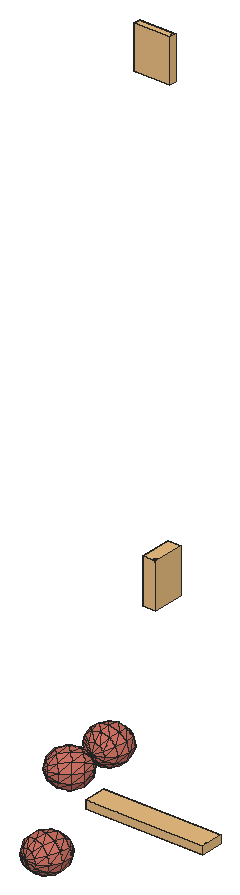
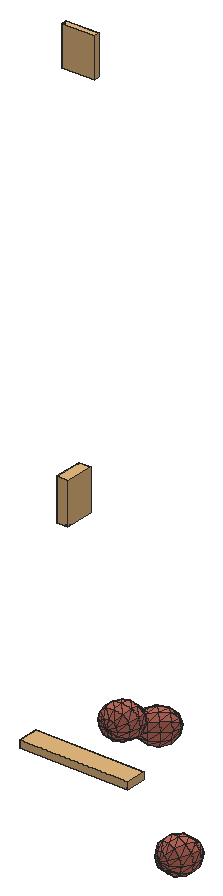
# SketchUp Ruby script. Lengths in inches.
U = 1.inch
M = Sketchup.active_model
def pt(a) = Geom::Point3d.new(a.map { |v| v * U })
def face(e, loops, mat)
  f = e.add_face(loops[0].map { |a| pt(a) })
  loops[1..].each { |l| e.add_face(l.map { |a| pt(a) }).erase! }
  f.material = f.back_material = mat if mat
  f
end
# faces: each face lists its corners as indices into pts; further lists are holes
def faces(e, pts, list, mat = nil) = list.each { |f| face(e, (f[0].is_a?(Array) ? f : [f]).map { |l| l.map { |i| pts[i] } }, mat) }
# xy, xz, yz: faces in a plane at the given z, y or x. An outline is a flat list of corners, or four numbers for a rectangle; further outlines are holes
def ring(l) = l.size == 4 ? [[l[0], l[1]], [l[2], l[1]], [l[2], l[3]], [l[0], l[3]]] : l.each_slice(2).to_a
def flat(e, list, mat, &to3) = list.each { |f| face(e, (f[0].is_a?(Array) ? f : [f]).map { |l| ring(l).map { |u, v| to3.(u, v) } }, mat) }
def xy(e, z, list, mat = nil) = flat(e, list, mat) { |x, y| [x, y, z] }
def xz(e, y, list, mat = nil) = flat(e, list, mat) { |x, z| [x, y, z] }
def yz(e, x, list, mat = nil) = flat(e, list, mat) { |y, z| [x, y, z] }
def lines(e, pts, list) = list.each { |a, b| e.add_line(pt(pts[a]), pt(pts[b])) }
# prism: a flat outline (further loops are holes) pulled along v
def prism(e, loops, v, mat = nil)
  f = face(e, loops, mat); d = Geom::Vector3d.new(v.map { |x| x * U })
  f.pushpull(f.normal.samedirection?(d) ? d.length : -d.length)
end
def box(e, o, s, mat = nil) = prism(e, [[o, [o[0] + s[0], o[1], o[2]], [o[0] + s[0], o[1] + s[1], o[2]], [o[0], o[1] + s[1], o[2]]]], [0, 0, s[2]], mat)
def at(x, y, z, deg = 0) = Geom::Transformation.translation(pt([x, y, z])) * Geom::Transformation.rotation(ORIGIN, Z_AXIS, deg.degrees)
def axes(o, x, y, z) = Geom::Transformation.new([*x, 0, *y, 0, *z, 0, *pt(o).to_a, 1])
def part(name) = M.definitions.add(name)
# library, detail: a bought-in or finely detailed component or shape, given as its bounding box
def library(name, o, s) = part(name).tap { |d| box(d.entities, o, s) }
def detail(e, o, s) = box(e.add_group.entities, o, s)
def put(e, d, t, mat = nil) = e.add_instance(d, t).tap { |i| i.material = mat if mat }
def group(e, t, mat = nil) = e.add_group.tap { |g| g.transformation = t; g.material = mat if mat }.entities
root = M.entities
M.materials.add("green").color = [174, 139, 102]
M.materials.add("vio").color = [206, 114, 100]
c1 = part("3DGeom~229_Defintion")
p = [[135.68,-61.63,-498.07],[-132.16,91.58,-492.59],[133.7,52.87,-500],[363.74,0,-373.43],[180.3,153.22,-454.61],[-51.45,265.375,-413.98],
  [185.71,-159.63,-449.34],[-128.73,-106.76,-489.25],[-362.61,105.75,-353.2],[-269.41,306.43,-262.42],[-269.41,306.43,-262.42],[-42.08,-276.49,-404.84],
  [-358.65,-123.27,-349.34],[262.99,212.5,-374.0625],[91.78,368.07,-274.47],[91.78,368.07,-274.47],[270.39,-214.85,-366.86],[-51.45,265.375,-413.98],
  [-269.41,306.43,-262.42],[-104.02,425.01,-101.32],[-51.45,265.375,-413.98],[91.78,368.07,-274.47],[104.59,-372.13,-261.99],[-258.59,-319.26,-251.875],
  [-42.08,-276.49,-404.84],[104.59,-372.13,-261.99],[-258.59,-319.26,-251.875],[359.62,214.85,-279.94],[262.99,212.5,-374.0625],[259.15,372.13,-111.44],
  [262.99,212.5,-374.0625],[259.15,372.13,-111.44],[359.62,214.85,-279.94],[367.02,-212.5,-272.74],[449.71,-153.21,-192.19],[367.02,-212.5,-272.74],
  [363.74,0,-373.43],[496.3125,-52.87,-146.8],[363.74,0,-373.43],[494.33,61.64,-148.73],[363.74,0,-373.43],[359.62,214.85,-279.94],
  [444.3,159.63,-197.46],[363.74,0,-373.43],[363.74,0,-373.43],[367.02,-212.5,-272.74],[104.59,-372.13,-261.99],[270.39,-214.85,-366.86],
  [-358.65,-123.27,-349.34],[-495.9,91.58,-119.16],[-362.61,105.75,-353.2],[-362.61,105.75,-353.2],[-415.1875,265.38,-40.55],[-362.61,105.75,-353.2],
  [-415.1875,265.38,-40.55],[-269.41,306.43,-262.42],[-258.59,-319.26,-251.875],[-492.47,-106.76,-115.82],[-358.65,-123.27,-349.34],[-358.65,-123.27,-349.34],
  [405.8125,276.49,31.41],[259.15,372.13,-111.44],[89.24,429.7,86.92],[259.15,372.13,-111.44],[367.02,-212.5,-272.74],[271.96,-368.07,-98.97],
  [104.59,-372.13,-261.99],[271.96,-368.07,-98.97],[367.02,-212.5,-272.74],[-415.1875,265.38,-40.55],[-271.96,368.07,98.97],[104.59,-372.13,-261.99],
  [-89.24,-429.7,-86.92],[-258.59,-319.26,-251.875],[104.59,-372.13,-261.99],[-405.8125,-276.49,-31.41],[-258.59,-319.26,-251.875],[-258.59,-319.26,-251.875],
  [-405.8125,-276.49,-31.41],[492.47,106.75,115.82],[415.1875,-265.375,40.55],[271.96,-368.07,-98.97],[495.9,-91.58,119.16],[-496.3125,52.87,146.8],
  [-449.71,153.21,192.19],[-415.1875,265.38,-40.55],[-494.33,-61.64,148.73],[259.15,372.13,-111.44],[258.59,319.26,251.875],[405.8125,276.49,31.41],
  [259.15,372.13,-111.44],[258.59,319.26,251.875],[-104.59,372.13,261.99],[104.02,-425.01,101.32],[415.1875,-265.375,40.55],[-259.15,-372.13,111.44],
  [-405.8125,-276.49,-31.41],[-415.1875,265.38,-40.55],[-367.02,212.5,272.74],[-415.1875,265.38,-40.55],[-367.02,212.5,272.74],[-271.96,368.07,98.97],
  [-259.15,-372.13,111.44],[-444.3,-159.63,197.46],[358.65,123.27,349.34],[258.59,319.26,251.875],[415.1875,-265.375,40.55],[269.41,-306.43,262.42],
  [269.41,-306.43,262.42],[42.08,276.49,404.84],[42.08,276.49,404.84],[258.59,319.26,251.875],[-367.02,212.5,272.74],[-270.39,214.85,366.86],
  [-270.39,214.85,366.86],[-91.78,-368.07,274.47],[-259.15,-372.13,111.44],[-359.62,-214.85,279.94],[-359.62,-214.85,279.94],[362.61,-105.75,353.2],
  [269.41,-306.43,262.42],[-363.74,0,373.43],[-367.02,212.5,272.74],[258.59,319.26,251.875],[42.08,276.49,404.84],[128.73,106.76,489.25],
  [258.59,319.26,251.875],[358.65,123.27,349.34],[-104.59,372.13,261.99],[-270.39,214.85,366.86],[-185.71,159.63,449.34],[-104.59,372.13,261.99],
  [51.45,-265.375,413.98],[362.61,-105.75,353.2],[51.45,-265.375,413.98],[269.41,-306.43,262.42],[-367.02,212.5,272.74],[-363.74,0,373.43],
  [-262.99,-212.5,374.0625],[-359.62,-214.85,279.94],[51.45,-265.375,413.98],[-262.99,-212.5,374.0625],[-91.78,-368.07,274.47],[-359.62,-214.85,279.94],
  [-262.99,-212.5,374.0625],[-363.74,0,373.43],[358.65,123.27,349.34],[132.16,-91.58,492.59],[362.61,-105.75,353.2],[358.65,123.27,349.34],
  [362.61,-105.75,353.2],[51.45,-265.375,413.98],[-363.74,0,373.43],[-262.99,-212.5,374.0625],[-180.3,-153.22,454.61],[-363.74,0,373.43],
  [-133.7,-52.87,500],[-363.74,0,373.43],[-135.68,61.63,498.07],[-363.74,0,373.43],[-363.74,0,373.43],[51.45,-265.375,413.98],
  [-262.99,-212.5,374.0625],[51.45,-265.375,413.98]]
faces(c1.entities,p,[[0,1,2],[0,2,3],[2,4,3],[2,1,5],[2,5,4],[6,7,0],[6,0,3],[0,7,1],
  [7,8,1],[1,8,9],[1,10,5],[11,12,7],[6,11,7],[7,12,8],[4,13,3],[4,5,14],
  [4,15,13],[16,11,6],[16,6,3],[17,18,19],[20,19,21],[22,23,24],[16,25,11],[11,26,12],
  [13,27,3],[28,21,29],[30,31,32],[33,16,3],[34,35,36],[37,34,38],[39,37,40],[41,42,43],
  [42,39,44],[45,46,47],[48,49,50],[51,49,52],[53,54,55],[56,57,58],[59,57,49],[41,60,42],
  [41,61,60],[21,19,62],[21,62,63],[64,65,66],[34,67,68],[18,69,70],[18,70,19],[71,72,73],
  [65,72,74],[72,75,76],[77,78,57],[42,79,39],[42,60,79],[34,80,81],[37,80,34],[39,79,82],
  [39,82,37],[37,82,80],[57,83,49],[49,83,84],[49,84,85],[78,86,57],[57,86,83],[87,88,89],
  [90,62,91],[19,70,92],[19,92,62],[65,93,72],[94,93,65],[72,95,96],[93,95,72],[97,84,98],
  [99,100,101],[102,103,78],[78,103,86],[60,104,79],[60,105,104],[106,107,93],[82,108,80],[62,92,109],
  [62,110,111],[70,112,113],[70,114,92],[93,115,95],[107,115,93],[116,117,103],[115,118,95],[79,104,119],
  [79,119,82],[82,119,120],[83,86,121],[84,83,121],[86,103,121],[122,84,121],[103,117,121],[123,124,125],
  [126,125,127],[128,129,130],[131,130,124],[107,132,115],[133,134,135],[129,136,137],[115,138,139],[140,141,142],
  [143,144,145],[146,147,148],[149,125,147],[150,147,151],[130,129,152],[153,154,155],[154,156,157],[156,158,159],
  [158,130,160],[161,154,162],[124,130,158],[124,158,125],[147,154,163],[147,156,154],[125,156,147],[125,158,156]],"vio")
c2 = library("3DGeom~19_Defintion",[-341.38,-500,-142.11],[682.76,1000,284.22])
c3 = part("3DGeom~20_Defintion")
p = [[-311.06,-487.18,-72.26],[-310.25,-484.5,-142.11],[-284.25,-498.77,-90.07],[-284.25,-498.77,-90.07],[-310.25,-484.5,-142.11],[-283.85,-497.43,-124.99],
  [-310.25,-484.5,-142.11],[-294.95,-491.76,-137.63],[-283.85,-497.43,-124.99],[-337.46,-474.24,-89.375],[-310.25,-484.5,-142.11],[-311.06,-487.18,-72.26],
  [-337.0625,-472.9,-124.3],[-310.25,-484.5,-142.11],[-337.46,-474.24,-89.375],[-310.25,-484.5,-142.11],[-337.0625,-472.9,-124.3],[-325.67,-477.6,-137.23],
  [-284.25,-498.77,-90.07],[-283.85,-497.43,-124.99],[-279.93,-500,-107.58],[-337.0625,-472.9,-124.3],[-337.46,-474.24,-89.375],[-341.38,-471.67,-106.78],
  [-311.06,-487.18,-72.26],[-284.25,-498.77,-90.07],[-295.64,-494.08,-77.14],[-337.46,-474.24,-89.375],[-311.06,-487.18,-72.26],[-326.37,-479.92,-76.74],
  [319.0625,494.74,82.9],[301.91,466.72,142.11],[318.42,461.52,137.94],[319.0625,494.74,82.9],[318.42,461.52,137.94],[332.8,461.46,126.96],
  [319.0625,494.74,82.9],[332.8,461.46,126.96],[341.21,466.57,112.1],[319.0625,494.74,82.9],[341.21,466.57,112.1],[341.38,475.47,97.35],
  [319.0625,494.74,82.9],[287.69,475.68,138.34],[301.91,466.72,142.11],[319.0625,494.74,82.9],[341.38,475.47,97.35],[333.27,485.79,86.67],
  [319.0625,494.74,82.9],[279.59,485.99,127.65],[287.69,475.68,138.34],[319.0625,494.74,82.9],[279.76,494.89,112.9],[279.59,485.99,127.65],
  [319.0625,494.74,82.9],[288.17,500,98.05],[279.76,494.89,112.9],[319.0625,494.74,82.9],[302.55,499.95,87.06],[288.17,500,98.05]]
faces(c3.entities,p,[[0,1,2],[3,4,5],[6,7,8],[9,10,11],[12,13,14],[15,16,17],[18,19,20],[21,22,23],
  [24,25,26],[27,28,29],[30,31,32],[33,34,35],[36,37,38],[39,40,41],[42,43,44],[45,46,47],
  [48,49,50],[51,52,53],[54,55,56],[57,58,59]],"green")
c4 = part("3DGeom~196_Defintion")
p = [[141.97,-189.5,-442.47],[-141.24,0,-495.8],[125.58,0,-500],[368.22,-109.41,-337.01],[368.22,-109.41,-337.01],[358.76,0,-370.22],
  [-122.32,218.8125,-429.38],[141.97,189.5,-442.47],[358.76,0,-370.22],[-122.32,-218.81,-429.38],[-370.22,0,-358.76],[-353.83,189.5,-301.23],
  [186.74,-328.22,-285.3125],[394.07,-189.5,-246.27],[394.07,-189.5,-246.27],[368.22,-109.41,-337.01],[358.76,0,-370.22],[368.22,109.41,-337.01],
  [368.22,109.41,-337.01],[186.74,328.22,-285.3125],[-70.62,378.99,-247.9],[-70.62,378.99,-247.9],[186.74,328.22,-285.3125],[-70.62,-378.99,-247.9],
  [-353.83,-189.5,-301.23],[-309.0625,328.22,-144.07],[-309.0625,328.22,-144.07],[-70.62,378.99,-247.9],[368.22,-109.41,-337.01],[358.76,0,-370.22],
  [495.8,0,-141.24],[368.22,109.41,-337.01],[-353.83,-189.5,-301.23],[-500,0,-125.58],[-370.22,0,-358.76],[-370.22,0,-358.76],
  [-490.54,109.41,-92.37],[-370.22,0,-358.76],[-353.83,189.5,-301.23],[394.07,-189.5,-246.27],[394.07,189.5,-246.27],[368.22,109.41,-337.01],
  [186.74,328.22,-285.3125],[394.07,189.5,-246.27],[-309.0625,-328.22,-144.07],[-309.0625,-328.22,-144.07],[-490.54,-109.41,-92.37],[-353.83,-189.5,-301.23],
  [-353.83,-189.5,-301.23],[-353.83,189.5,-301.23],[-464.6875,189.5,-1.63],[-353.83,189.5,-301.23],[-309.0625,328.22,-144.07],[247.9,-378.99,-70.62],
  [-70.62,-378.99,-247.9],[186.74,-328.22,-285.3125],[429.38,-218.8125,-122.32],[247.9,-378.99,-70.62],[186.74,-328.22,-285.3125],[186.74,-328.22,-285.3125],
  [186.74,328.22,-285.3125],[247.9,378.99,-70.62],[186.74,328.22,-285.3125],[-70.62,378.99,-247.9],[0,437.625,0],[186.74,328.22,-285.3125],
  [247.9,378.99,-70.62],[0,-437.625,0],[-309.0625,-328.22,-144.07],[-70.62,-378.99,-247.9],[247.9,-378.99,-70.62],[-70.62,-378.99,-247.9],
  [-309.0625,328.22,-144.07],[-247.9,378.99,70.62],[429.38,218.8125,-122.32],[-247.9,-378.99,70.62],[-309.0625,-328.22,-144.07],[-247.9,-378.99,70.62],
  [-464.6875,-189.5,-1.63],[-309.0625,-328.22,-144.07],[-309.0625,-328.22,-144.07],[-309.0625,328.22,-144.07],[-429.38,218.8125,122.32],[-309.0625,328.22,-144.07],
  [-247.9,378.99,70.62],[464.6875,-189.5,1.63],[490.54,-109.41,92.37],[500,0,125.58],[464.6875,189.5,1.63],[490.54,109.41,92.37],
  [-495.8,0,141.24],[309.0625,328.22,144.07],[309.0625,-328.22,144.07],[247.9,-378.99,-70.62],[309.0625,-328.22,144.07],[247.9,378.99,-70.62],
  [70.62,378.99,247.9],[309.0625,328.22,144.07],[247.9,378.99,-70.62],[70.62,378.99,247.9],[-247.9,-378.99,70.62],[-429.38,-218.8125,122.32],
  [70.62,-378.99,247.9],[309.0625,-328.22,144.07],[-186.74,328.22,285.3125],[-186.74,328.22,285.3125],[70.62,378.99,247.9],[353.83,189.5,301.23],
  [-186.74,-328.22,285.3125],[-247.9,-378.99,70.62],[-186.74,-328.22,285.3125],[-247.9,378.99,70.62],[-394.07,189.5,246.27],[-247.9,378.99,70.62],
  [-394.07,189.5,246.27],[-186.74,328.22,285.3125],[353.83,-189.5,301.23],[370.22,0,358.76],[-186.74,-328.22,285.3125],[-394.07,-189.5,246.27],
  [-394.07,189.5,246.27],[-368.22,-109.41,337.01],[-368.22,-109.41,337.01],[-358.76,0,370.22],[-358.76,0,370.22],[-368.22,109.41,337.01],
  [-368.22,109.41,337.01],[-394.07,189.5,246.27],[353.83,-189.5,301.23],[70.62,-378.99,247.9],[309.0625,-328.22,144.07],[309.0625,328.22,144.07],
  [122.32,218.8125,429.38],[353.83,189.5,301.23],[309.0625,328.22,144.07],[70.62,378.99,247.9],[-141.97,-189.5,442.47],[-394.07,-189.5,246.27],
  [-186.74,-328.22,285.3125],[-368.22,-109.41,337.01],[-394.07,-189.5,246.27],[-186.74,328.22,285.3125],[-394.07,189.5,246.27],[-368.22,109.41,337.01],
  [122.32,-218.8125,429.38],[-186.74,-328.22,285.3125],[70.62,-378.99,247.9],[353.83,-189.5,301.23],[70.62,-378.99,247.9],[-141.97,189.5,442.47],
  [-186.74,-328.22,285.3125],[370.22,0,358.76],[353.83,-189.5,301.23],[353.83,189.5,301.23],[141.24,0,495.8],[353.83,189.5,301.23],
  [370.22,0,358.76],[-125.58,0,500],[-358.76,0,370.22],[370.22,0,358.76]]
faces(c4.entities,p,[[0,1,2],[3,0,2],[4,2,5],[2,1,6],[2,6,7],[8,2,7],[9,10,1],[0,9,1],
  [1,10,11],[1,11,6],[12,9,0],[13,12,0],[14,0,15],[16,7,17],[18,7,19],[7,6,20],
  [7,21,22],[23,24,9],[12,23,9],[9,24,10],[6,11,25],[6,26,27],[28,29,30],[29,31,30],
  [32,33,34],[35,33,36],[37,36,38],[39,28,30],[31,40,30],[41,42,43],[23,44,24],[45,46,47],
  [48,46,33],[49,36,50],[51,50,52],[53,54,55],[56,57,58],[56,59,39],[40,60,61],[62,63,64],
  [65,64,66],[67,68,69],[70,67,71],[63,72,73],[63,73,64],[56,39,30],[40,74,30],[40,61,74],
  [67,75,76],[77,78,79],[80,78,46],[81,50,82],[83,82,84],[85,56,30],[86,85,30],[87,86,30],
  [74,88,30],[88,89,30],[89,87,30],[33,46,90],[36,33,90],[85,57,56],[74,91,88],[74,61,91],
  [46,78,90],[50,36,90],[92,67,93],[85,94,57],[95,96,97],[98,64,99],[100,101,78],[78,101,90],
  [82,50,90],[102,75,67],[103,102,67],[64,73,104],[64,105,106],[86,94,85],[88,107,89],[88,91,107],
  [108,101,109],[102,110,75],[111,82,112],[113,114,115],[86,116,94],[87,116,86],[89,107,117],[89,117,87],
  [118,119,101],[101,119,90],[120,82,90],[87,117,116],[119,121,90],[122,123,90],[124,125,90],[126,127,90],
  [128,129,130],[131,132,133],[134,135,132],[136,137,138],[136,139,140],[141,142,143],[144,145,146],[147,144,148],
  [135,141,149],[135,149,132],[144,136,150],[141,143,149],[151,144,152],[153,132,154],[155,154,156],[157,139,136],
  [157,158,139],[149,143,158],[159,154,144],[149,158,157],[154,136,144],[132,149,157],[132,157,154],[154,157,136]],"vio")
c5 = library("3DGeom~27_Defintion",[-78.21,-500,-418.56],[156.42,1000,837.12])
c6 = part("3DGeom~28_Defintion")
p = [[46.32,-458.84,-418.56],[37.22,-500,-363.86],[12.49,-468.47,-409.44],[75.6,-469.79,-400.32],[37.22,-500,-363.86],[75.6,-469.79,-400.32],
  [63.93,-461.98,-412.26],[12.49,-468.47,-409.44],[27.49,-461.21,-417.52],[12.49,-468.47,-409.44],[37.22,-500,-363.86],[7.94,-489.05,-382.09],
  [12.49,-468.47,-409.44],[7.94,-489.05,-382.09],[5.33,-478.66,-396.47],[71.06,-490.37,-372.98],[37.22,-500,-363.86],[75.6,-469.79,-400.32],
  [71.06,-490.37,-372.98],[75.6,-469.79,-400.32],[78.21,-480.18,-385.94],[37.22,-500,-363.86],[19.61,-496.86,-370.16],[7.94,-489.05,-382.09],
  [37.22,-500,-363.86],[71.06,-490.37,-372.98],[56.05,-497.625,-364.89],[-47.11,487.39,418.56],[-36.4375,500,347.21],[-55.37,499.54,349.35],
  [-47.11,487.39,418.56],[-18.93,498.77,354.62],[-36.4375,500,347.21],[-47.11,487.39,418.56],[-55.37,499.54,349.35],[-70.66,497.51,360.48],
  [-47.11,487.39,418.56],[-7.55,496.1875,369.6],[-18.93,498.77,354.62],[-47.11,487.39,418.56],[-70.66,497.51,360.48],[-78.21,494.45,377.62],
  [-47.11,487.39,418.56],[-5.33,492.93,388.15],[-7.55,496.1875,369.6],[-47.11,487.39,418.56],[-78.21,494.45,377.62],[-76,491.2,396.16],
  [-47.11,487.39,418.56],[-12.88,489.88,405.28],[-5.33,492.93,388.15],[-47.11,487.39,418.56],[-76,491.2,396.16],[-64.61,488.61,411.15],
  [-47.11,487.39,418.56],[-28.17,487.85,416.41],[-12.88,489.88,405.28]]
faces(c6.entities,p,[[0,1,2],[3,4,0],[5,0,6],[0,7,8],[9,10,11],[12,13,14],[15,16,17],[18,19,20],
  [21,22,23],[24,25,26],[27,28,29],[30,31,32],[33,34,35],[36,37,38],[39,40,41],[42,43,44],
  [45,46,47],[48,49,50],[51,52,53],[54,55,56]],"green")
c7 = library("3DGeom~15_Defintion",[-93.43,-35.39,-500],[186.86,70.78,1000])
c8 = part("3DGeom~16_Defintion")
p = [[-67.78,-34.5625,-497.5],[-75.6,-25.33,-500],[-54.89,-33.15,-493.42],[-75.6,-25.33,-500],[-67.78,-34.5625,-497.5],[-73.08,-30.88,-499.18],
  [-54.89,-33.15,-493.42],[-75.6,-25.33,-500],[-49.81,-22.5,-491.85],[-75.6,-25.33,-500],[-74.66,-19.4,-499.72],[-70.52,-14.68,-498.43],
  [-57.625,-13.26,-494.36],[-75.6,-25.33,-500],[-70.52,-14.68,-498.43],[-49.81,-22.5,-491.85],[-75.6,-25.33,-500],[-57.625,-13.26,-494.36],
  [-57.625,-13.26,-494.36],[-70.52,-14.68,-498.43],[-64.28,-12.43,-496.47],[-67.78,-34.5625,-497.5],[-54.89,-33.15,-493.42],[-61.125,-35.39,-495.39],
  [-49.81,-22.5,-491.85],[-57.625,-13.26,-494.36],[-52.33,-16.95,-492.67],[-54.89,-33.15,-493.42],[-49.81,-22.5,-491.85],[-50.75,-28.42,-492.13],
  [67.2,22.73,500],[92.46,19.2,493.88],[93.43,25.1,493.15],[67.2,22.73,500],[93.43,25.1,493.15],[90.88,30.68,493.34],
  [67.2,22.73,500],[90.88,30.68,493.34],[85.51,34.45,494.39],[67.2,22.73,500],[88.24,14.5625,495.33],[92.46,19.2,493.88],
  [67.2,22.73,500],[85.51,34.45,494.39],[78.74,35.39,496.03],[67.2,22.73,500],[81.9,12.43,497.11],[88.24,14.5625,495.33],
  [67.2,22.73,500],[78.74,35.39,496.03],[72.39,33.26,497.82],[67.2,22.73,500],[75.13,13.38,498.76],[81.9,12.43,497.11],
  [67.2,22.73,500],[72.39,33.26,497.82],[68.17,28.625,499.27],[67.2,22.73,500],[69.75,17.15,499.8125],[75.13,13.38,498.76]]
faces(c8.entities,p,[[0,1,2],[3,4,5],[6,7,8],[9,10,11],[12,13,14],[15,16,17],[18,19,20],[21,22,23],
  [24,25,26],[27,28,29],[30,31,32],[33,34,35],[36,37,38],[39,40,41],[42,43,44],[45,46,47],
  [48,49,50],[51,52,53],[54,55,56],[57,58,59]],"green")
c9 = part("3DGeom~188_Defintion")
p = [[-5.63,-212.24,-433.01],[-255.63,0,-429.76],[-6.51,0,-500],[245.12,-183.8,-378.25],[244.37,0,-436.27],[-254.88,183.8,-371.75],
  [-5.63,212.24,-433.01],[430.2,-106.12,-222.14],[430.2,-106.12,-222.14],[429.76,0,-255.63],[245.12,183.8,-378.25],[429.76,0,-255.63],
  [245.12,183.8,-378.25],[-3.25,-367.61,-250],[-254.88,-183.8,-371.75],[247.18,-318.36,-219.76],[247.18,-318.36,-219.76],[-252.82,318.36,-213.25],
  [245.12,183.8,-378.25],[-3.25,367.61,-250],[-252.82,318.36,-213.25],[-3.25,367.61,-250],[-254.88,-183.8,-371.75],[-436.27,0,-244.37],
  [-255.63,0,-429.76],[-255.63,0,-429.76],[-435.83,106.12,-210.87],[-255.63,0,-429.76],[-254.88,183.8,-371.75],[431.39,-183.8,-130.63],
  [247.18,-318.36,-219.76],[245.12,-183.8,-378.25],[245.12,-183.8,-378.25],[430.2,-106.12,-222.14],[429.76,0,-255.63],[245.12,183.8,-378.25],
  [430.2,106.12,-222.14],[430.2,106.12,-222.14],[245.12,183.8,-378.25],[247.18,318.36,-219.76],[245.12,183.8,-378.25],[-3.25,367.61,-250],
  [247.18,318.36,-219.76],[-252.82,-318.36,-213.25],[-252.82,-318.36,-213.25],[-435.83,-106.12,-210.87],[-254.88,-183.8,-371.75],[-254.88,-183.8,-371.75],
  [-254.88,183.8,-371.75],[-434.64,183.8,-119.36],[-254.88,183.8,-371.75],[-252.82,318.36,-213.25],[429.76,0,-255.63],[500,0,-6.51],
  [0,-424.48,0],[-252.82,-318.36,-213.25],[-3.25,-367.61,-250],[250,-367.61,-3.25],[-3.25,-367.61,-250],[250,-367.61,-3.25],
  [-3.25,-367.61,-250],[247.18,-318.36,-219.76],[-3.25,367.61,-250],[-252.82,318.36,-213.25],[-250,367.61,3.25],[247.18,318.36,-219.76],
  [0,424.48,0],[-500,0,6.51],[431.39,183.8,-130.63],[433.01,-212.24,-5.63],[250,-367.61,-3.25],[250,367.61,-3.25],
  [247.18,318.36,-219.76],[250,367.61,-3.25],[-250,-367.61,3.25],[-252.82,-318.36,-213.25],[-250,-367.61,3.25],[-434.64,-183.8,-119.37],
  [-252.82,-318.36,-213.25],[-252.82,-318.36,-213.25],[-252.82,318.36,-213.25],[-433.01,212.24,5.63],[-252.82,318.36,-213.25],[-250,367.61,3.25],
  [433.01,212.24,-5.63],[-250,-367.61,3.25],[-433.01,-212.24,5.63],[434.64,-183.8,119.37],[435.83,-106.12,210.87],[436.27,0,244.37],
  [434.64,183.8,119.37],[435.83,106.12,210.87],[252.82,318.36,213.25],[252.82,-318.36,213.25],[250,-367.61,-3.25],[252.82,-318.36,213.25],
  [250,367.61,-3.25],[3.25,367.61,250],[252.82,318.36,213.25],[250,367.61,-3.25],[3.25,367.61,250],[3.25,-367.61,250],
  [252.82,-318.36,213.25],[-247.18,318.36,219.76],[-247.18,318.36,219.76],[3.25,367.61,250],[-247.18,-318.36,219.76],[-250,-367.61,3.25],
  [-247.18,-318.36,219.76],[-250,367.61,3.25],[-431.39,183.8,130.63],[-250,367.61,3.25],[-247.18,318.36,219.76],[-247.18,-318.36,219.76],
  [-431.39,-183.8,130.63],[-430.2,-106.12,222.14],[-429.76,0,255.63],[-429.76,0,255.63],[-430.2,106.12,222.14],[-430.2,106.12,222.14],
  [254.88,183.8,371.75],[-245.12,-183.8,378.25],[-247.18,-318.36,219.76],[-245.12,-183.8,378.25],[-247.18,318.36,219.76],[-430.2,106.12,222.14],
  [254.88,-183.8,371.75],[255.63,0,429.76],[254.88,-183.8,371.75],[3.25,-367.61,250],[252.82,-318.36,213.25],[252.82,318.36,213.25],
  [5.63,212.24,433.01],[254.88,183.8,371.75],[252.82,318.36,213.25],[3.25,367.61,250],[5.63,-212.24,433.01],[-247.18,-318.36,219.76],
  [3.25,-367.61,250],[-245.12,-183.8,378.25],[-247.18,-318.36,219.76],[-247.18,318.36,219.76],[-430.2,106.12,222.14],[-245.12,183.8,378.25],
  [-247.18,318.36,219.76],[-245.12,183.8,378.25],[-244.37,0,436.27],[-430.2,-106.12,222.14],[-429.76,0,255.63],[-430.2,-106.12,222.14],
  [-430.2,106.12,222.14],[254.88,-183.8,371.75],[3.25,-367.61,250],[255.63,0,429.76],[254.88,-183.8,371.75],[254.88,183.8,371.75],
  [6.51,0,500],[254.88,183.8,371.75],[255.63,0,429.76],[255.63,0,429.76]]
faces(c9.entities,p,[[0,1,2],[3,0,2],[3,2,4],[2,1,5],[2,5,6],[4,2,6],[7,3,4],[8,4,9],
  [4,6,10],[11,4,12],[13,14,0],[15,13,0],[16,0,3],[0,14,1],[6,5,17],[18,6,19],
  [6,20,21],[22,23,24],[25,23,26],[27,26,28],[29,30,31],[29,32,33],[34,35,36],[37,38,39],
  [40,41,42],[13,43,14],[44,45,46],[47,45,23],[48,26,49],[50,49,51],[33,52,53],[52,37,53],
  [54,55,56],[57,54,58],[59,60,61],[62,63,64],[65,62,66],[62,64,66],[23,45,67],[26,23,67],
  [29,33,53],[37,68,53],[37,39,68],[69,70,30],[69,30,29],[68,39,71],[72,66,73],[54,74,75],
  [76,77,78],[79,77,45],[80,49,81],[82,81,83],[45,77,67],[49,26,67],[69,29,53],[68,84,53],
  [68,71,84],[85,86,77],[77,86,67],[81,49,67],[87,69,53],[88,87,53],[89,88,53],[84,90,53],
  [90,91,53],[91,89,53],[87,70,69],[84,92,90],[84,71,92],[93,54,94],[87,95,70],[96,97,98],
  [99,66,100],[101,74,54],[102,101,54],[66,64,103],[66,104,105],[106,86,107],[101,108,74],[109,81,110],
  [111,110,112],[113,114,86],[86,114,67],[110,81,67],[114,115,67],[115,116,67],[117,118,67],[119,110,67],
  [88,95,87],[90,120,91],[90,92,120],[121,114,122],[123,115,114],[124,110,125],[88,126,95],[89,126,88],
  [91,120,127],[91,127,89],[128,129,130],[131,132,133],[134,135,132],[136,137,138],[136,139,140],[141,142,143],
  [135,144,145],[146,147,139],[146,148,149],[145,150,148],[89,127,126],[151,136,152],[135,145,132],[145,148,146],
  [153,136,154],[155,132,156],[157,156,158],[156,139,136],[156,146,139],[132,145,146],[159,156,136],[132,146,156]],"vio")
g1 = group(root,at(15.3125,38.42,26.21))
put(g1,c1,axes([2.4375,-0.15,10.98],[0,0.00037,0],[0,0,-0.00037],[-0.00037,0,0]),"vio")
g2 = group(root,at(15.3125,38.42,26.21))
put(g2,c2,axes([3.24,-0.08,12.83],[0,0.00042,0],[0,0,-0.00042],[-0.00042,0,0]),"green")
put(g2,c3,axes([3.24,-0.08,12.83],[0,0.00042,0],[0,0,-0.00042],[-0.00042,0,0]),"green")
g3 = group(root,at(15.3125,38.42,26.21))
put(g3,c4,axes([2.05,0.07,10.04],[0,0.00038,0],[0,0,-0.00038],[-0.00038,0,0]),"vio")
g4 = group(root,at(15.3125,38.42,26.21))
put(g4,c5,axes([3.02,0.11,17.03],[0,0.0004,0],[0,0,-0.0004],[-0.0004,0,0]),"green")
put(g4,c6,axes([3.02,0.11,17.03],[0,0.0004,0],[0,0,-0.0004],[-0.0004,0,0]),"green")
g5 = group(root,at(15.3125,38.42,26.21))
put(g5,c7,axes([2.99,0.13,10.6],[0,0.00109,0],[0,0,-0.00109],[-0.00109,0,0]),"green")
put(g5,c8,axes([2.99,0.13,10.6],[0,0.00109,0],[0,0,-0.00109],[-0.00109,0,0]),"green")
g6 = group(root,at(15.3125,38.42,26.21))
put(g6,c9,axes([2.58,0.13,11.1],[0,0.00039,0],[0,0,-0.00039],[-0.00039,0,0]),"vio")
